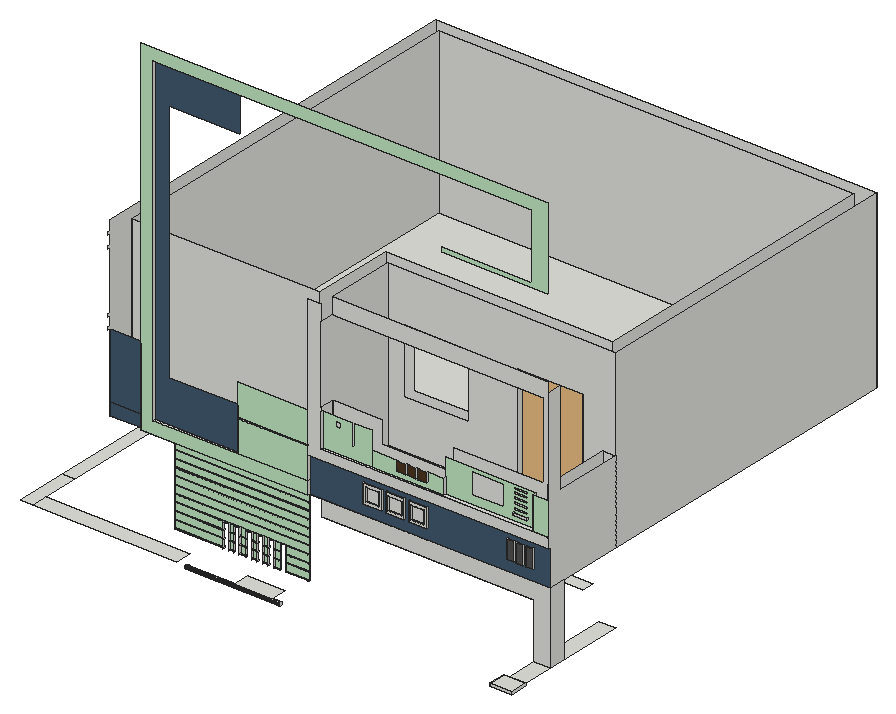
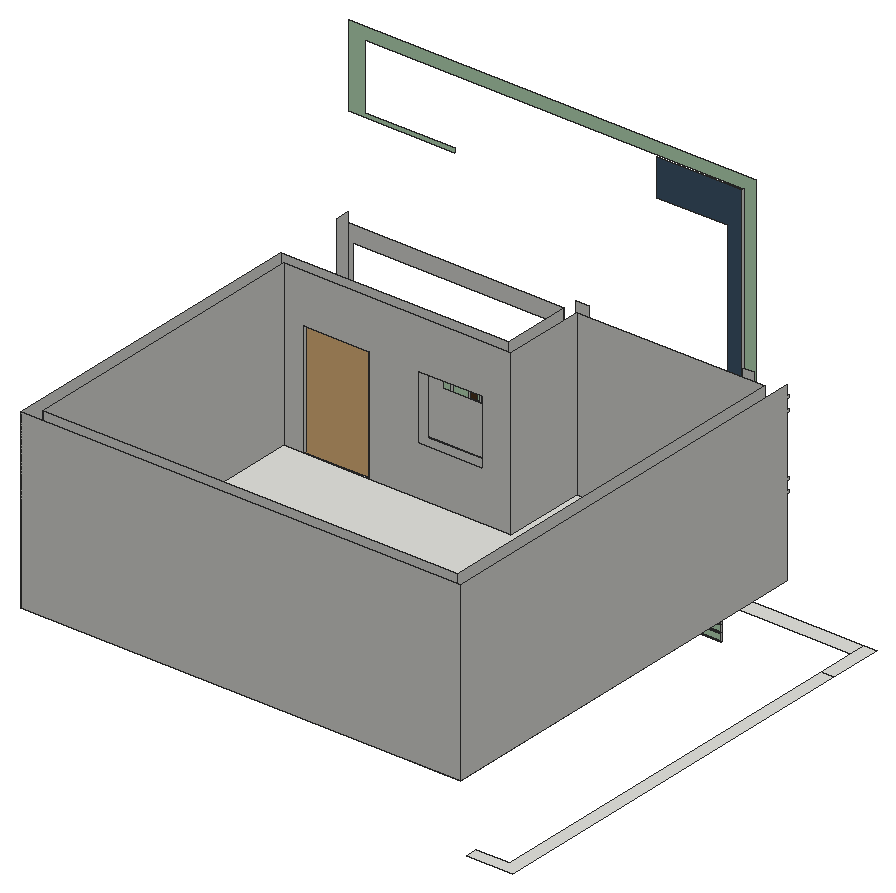
# SketchUp Ruby script. Lengths in inches.
U = 1.inch
M = Sketchup.active_model
def pt(a) = Geom::Point3d.new(a.map { |v| v * U })
def face(e, loops, mat)
  f = e.add_face(loops[0].map { |a| pt(a) })
  loops[1..].each { |l| e.add_face(l.map { |a| pt(a) }).erase! }
  f.material = f.back_material = mat if mat
  f
end
# faces: each face lists its corners as indices into pts; further lists are holes
def faces(e, pts, list, mat = nil) = list.each { |f| face(e, (f[0].is_a?(Array) ? f : [f]).map { |l| l.map { |i| pts[i] } }, mat) }
# xy, xz, yz: faces in a plane at the given z, y or x. An outline is a flat list of corners, or four numbers for a rectangle; further outlines are holes
def ring(l) = l.size == 4 ? [[l[0], l[1]], [l[2], l[1]], [l[2], l[3]], [l[0], l[3]]] : l.each_slice(2).to_a
def flat(e, list, mat, &to3) = list.each { |f| face(e, (f[0].is_a?(Array) ? f : [f]).map { |l| ring(l).map { |u, v| to3.(u, v) } }, mat) }
def xy(e, z, list, mat = nil) = flat(e, list, mat) { |x, y| [x, y, z] }
def xz(e, y, list, mat = nil) = flat(e, list, mat) { |x, z| [x, y, z] }
def yz(e, x, list, mat = nil) = flat(e, list, mat) { |y, z| [x, y, z] }
def lines(e, pts, list) = list.each { |a, b| e.add_line(pt(pts[a]), pt(pts[b])) }
# prism: a flat outline (further loops are holes) pulled along v
def prism(e, loops, v, mat = nil)
  f = face(e, loops, mat); d = Geom::Vector3d.new(v.map { |x| x * U })
  f.pushpull(f.normal.samedirection?(d) ? d.length : -d.length)
end
def box(e, o, s, mat = nil) = prism(e, [[o, [o[0] + s[0], o[1], o[2]], [o[0] + s[0], o[1] + s[1], o[2]], [o[0], o[1] + s[1], o[2]]]], [0, 0, s[2]], mat)
def at(x, y, z, deg = 0) = Geom::Transformation.translation(pt([x, y, z])) * Geom::Transformation.rotation(ORIGIN, Z_AXIS, deg.degrees)
def axes(o, x, y, z) = Geom::Transformation.new([*x, 0, *y, 0, *z, 0, *pt(o).to_a, 1])
def part(name) = M.definitions.add(name)
# library, detail: a bought-in or finely detailed component or shape, given as its bounding box
def library(name, o, s) = part(name).tap { |d| box(d.entities, o, s) }
def detail(e, o, s) = box(e.add_group.entities, o, s)
def put(e, d, t, mat = nil) = e.add_instance(d, t).tap { |i| i.material = mat if mat }
def group(e, t, mat = nil) = e.add_group.tap { |g| g.transformation = t; g.material = mat if mat }.entities
root = M.entities
M.materials.add("Teddy_SkinShadow ").color = [76, 52, 30]
M.materials.add("[0111_SlateGray]").color = [66, 89, 112]
M.materials.add("[0116_Lavender]").color = [195, 232, 195]
M.materials.add("[0135_DarkGray]1").color = [81, 81, 81]
c1 = library("porta 4",[0.2,-5.42,1.33],[46.55,4.72,83.21])
xy(root,62.5,[[131.18,38.4375,135.87,39],[83,38.5,119.37,39],[140.12,38.5,144.12,39],[148.37,38.5,152.12,39],[156.37,38.5,160.62,39],
  [164.87,38.5,182,39],[123.62,38.625,126.93,39]])
xy(root,63.25,[[83,38.5,119.37,39],[131.18,38.5,135.87,39],[140.12,38.5,144.12,39],[148.37,38.5,152.12,39],[156.37,38.5,160.62,39],
  [164.87,38.5,182,39],[123.62,38.625,126.93,39]])
xy(root,67,[[345,1,361,3],[345,3,347,12],[347,3,359,14],[359,3,361,14],[345,12,347,14],
  [347,14,359,39],[347,51,359,99]])
xy(root,68.25,[[83,38.5,119.37,39],[131.18,38.5,135.87,39],[140.12,38.5,144.12,39],[148.37,38.5,152.12,39],[156.37,38.5,160.62,39],
  [164.87,38.5,182,39],[123.62,38.625,126.93,39]])
xy(root,69,[[0,0,9,39],[9,0,115.21,12],[157.75,0,185.01,12],[345,1,361,14],[83,38.5,119.37,39],
  [131.18,38.5,135.87,39],[140.12,38.5,144.12,39],[148.37,38.5,152.12,39],[156.37,38.5,160.62,39],[164.87,38.5,182,39],
  [123.62,38.625,126.93,39],[0,39,9,39,9,325.8,34,325.8,34,334.8,0,334.8]])
xy(root,74,[[83,38.5,119.37,39],[131.18,38.5,135.87,39],[140.12,38.5,144.12,39],[148.37,38.5,152.12,39],[156.37,38.5,160.62,39],
  [164.87,38.5,182,39],[123.62,38.625,126.93,39]])
xy(root,74.75,[[83,38.5,119.37,39],[123.62,38.5,126.93,39],[131.18,38.5,135.87,39],[140.12,38.5,144.12,39],[148.37,38.5,152.12,39],
  [156.37,38.5,160.62,39],[164.87,38.5,182,39]])
xy(root,79.75,[[83,38.5,119.37,39],[164.87,38.5,182,39]])
xy(root,80.25,[[126.93,37.375,131.18,39],[135.87,37.4375,140.12,39],[144.12,37.4375,148.37,39],[119.37,37.5625,123.62,39],[152.12,37.875,156.37,39],
  [123.62,38.5,126.93,39],[131.18,38.5,135.87,39],[140.12,38.5,144.12,39],[148.37,38.5,152.12,39],[156.37,38.5,160.62,39]])
xy(root,80.5,[[83,38.5,119.37,39],[119.37,38.5,164.87,39],[164.87,38.5,182,39]])
xy(root,84,[[203,99,251,108],[287,99,335,108]])
xy(root,85.5,[[83,38.5,119.37,39],[119.37,38.5,164.87,39],[164.87,38.5,182,39]])
xy(root,86.25,[[83,38.5,119.37,39],[119.37,38.5,164.87,39],[164.87,38.5,182,39]])
xy(root,91.25,[[83,38.5,119.37,39],[119.37,38.5,164.87,39],[164.87,38.5,182,39]])
xy(root,92,[[83,38.5,119.37,39],[119.37,38.5,164.87,39],[164.87,38.5,182,39]])
xy(root,97,[[83,38.5,119.37,39],[119.37,38.5,164.87,39],[164.87,38.5,182,39]])
xy(root,97.75,[[83,38.5,119.37,39],[119.37,38.5,164.87,39],[164.87,38.5,182,39]])
xy(root,102.75,[[83,38.5,119.37,39],[119.37,38.5,164.87,39],[164.87,38.5,182,39]])
xy(root,103.5,[[83,38.5,119.37,39],[119.37,38.5,164.87,39],[164.87,38.5,182,39]])
xy(root,108,[[191,39,347,51]])
xy(root,108.5,[[83,38.5,119.37,39],[119.37,38.5,164.87,39],[164.87,38.5,182,39]])
xy(root,109.25,[[83,38.5,119.37,39],[119.37,38.5,164.87,39],[164.87,38.5,182,39]])
xy(root,114.25,[[83,38.5,119.37,39],[119.37,38.5,164.87,39],[164.87,38.5,182,39]])
xy(root,115,[[83,38.5,119.37,39],[119.37,38.5,164.87,39],[164.87,38.5,182,39]])
xy(root,120,[[59,37,59,39,83,39,83,38.5,182,38.5,182,37],[83,38.5,182,39],[35,39,44,339],[44,39,83,48],[83,39,92,99],
  [92,39,92,48,182,48,182,90,92,90,92,99,191,99,191,39],[191,39,359,51],[44,48,83,330],[92,48,182,90],[191,51,359,99],
  [83,99,92,108],[92,99,359,99,359,339,92,339,92,330,350,330,350,108,92,108],[83,108,92,339],[92,108,350,330],[44,330,83,339]])
xy(root,127.88,[[221.83,38,235.58,39],[238.46,38,252.21,39],[255.27,38,269.02,39]])
xy(root,128.49,[[327.94,38,332.88,39],[334.69,38,339.63,39],[342,38,346.94,39]])
xy(root,129,[[68,37,182,37,182,37.5,130.11,37.5,130.11,39,68,39],[130.11,37.5,182,39],[44,48,182.375,48,182.375,108,350,108,350,330,44,330],[191.375,48,350,48,350,99,334.8125,99,334.8125,108,287,108,287,99,191.375,99]])
xy(root,129.88,[[223.83,38,233.58,39],[240.46,38,250.21,39],[257.27,38,267.02,39]])
xy(root,139.63,[[223.83,38,233.58,39],[240.46,38,250.21,39],[257.27,38,267.02,39]])
xy(root,141.63,[[221.83,38,235.58,39],[238.46,38,252.21,39],[255.27,38,269.02,39]])
xy(root,141.87,[[327.94,38,332.88,39],[334.69,38,339.63,39],[342,38,346.94,39]])
xy(root,146.25,[[182,37.5,359,39]])
xy(root,152,[[130.11,37.5,182,39]])
xy(root,153,[[130.11,37.5,182,39]])
xy(root,153.78,[[191.375,37.5,227.375,39],[227.375,37.5,280.75,39],[280.75,37.5,359,37.5,359,38,347,38,347,40.75,280.75,40.75]])
xy(root,157.71,[[330.79,39.75,341.29,40.75]])
xy(root,158.06,[[247.03,38,253.34,39],[254.72,38,261.03,39],[262.4,38,268.72,39]])
xz(root,1,[[345,67,361,69]])
xz(root,14,[[345,67,361,69]])
xz(root,37,[[59,120,182,120,182,129,68,129,68,366,347,366,347,318,280.59,318,280.59,315,359,315,359,375,59,375]],"[0116_Lavender]")
xz(root,37.5,[[182,146.25,359,146.25,359,153.78,191.375,153.78,191.375,249,182,249]])
xz(root,37.5,[[130.11,129,182,152],[130.11,153,182,176]],"[0116_Lavender]")
xz(root,38,[[[221.83,127.88,235.58,141.63],[223.83,129.88,233.58,139.63]],[[238.46,127.88,252.21,141.63],[240.46,129.88,250.21,139.63]],[[255.27,127.88,269.02,141.63],[257.27,129.88,267.02,139.63]]])
xz(root,38,[[247.03,158.06,253.34,164.72],[254.72,158.06,261.03,164.72],[262.4,158.06,268.72,164.72]],"Teddy_SkinShadow ")
xz(root,38,[[347,153.78,359,177.875]],"[0116_Lavender]")
xz(root,38,[[327.94,128.49,332.88,141.87],[334.69,128.49,339.63,141.87],[342,128.49,346.94,141.87]],"[0135_DarkGray]1")
xz(root,38.5,[[83,63.25,119.37,68.25],[131.18,63.25,135.87,68.25],[140.12,63.25,144.12,68.25],[148.37,63.25,152.12,68.25],[156.37,63.25,160.62,68.25],
  [164.87,63.25,182,68.25],[83,69,119.37,74],[131.18,69,135.87,74],[140.12,69,144.12,74],[148.37,69,152.12,74],
  [156.37,69,160.62,74],[164.87,69,182,74],[83,74.75,119.37,79.75],[123.62,74.75,126.93,80.25],[131.18,74.75,135.87,80.25],
  [140.12,74.75,144.12,80.25],[148.37,74.75,152.12,80.25],[156.37,74.75,160.62,80.25],[164.87,74.75,182,79.75],[83,80.5,182,85.5],
  [83,86.25,182,91.25],[83,92,182,97],[83,97.75,182,102.75],[83,103.5,182,108.5],[83,109.25,182,114.25],
  [83,115,182,120]],"[0116_Lavender]")
xz(root,38.625,[[123.62,63.25,126.93,68.25],[123.62,69,126.93,74]],"[0116_Lavender]")
xz(root,39,[[83,62.5,119.37,63.25],[123.62,62.5,126.93,63.25],[131.18,62.5,135.87,63.25],[140.12,62.5,144.12,63.25],[148.37,62.5,152.12,63.25],
  [156.37,62.5,160.62,63.25],[164.87,62.5,182,63.25],[347,67,359,67,359,120,191,120,191,108,347,108],[83,68.25,119.37,69],[123.62,68.25,126.93,69],
  [131.18,68.25,135.87,69],[140.12,68.25,144.12,69],[148.37,68.25,152.12,69],[156.37,68.25,160.62,69],[83,74,119.37,74.75],
  [123.62,74,126.93,74.75],[131.18,74,135.87,74.75],[140.12,74,144.12,74.75],[148.37,74,152.12,74.75],[156.37,74,160.62,74.75],
  [164.87,74,182,74.75],[83,79.75,119.37,79.75,119.37,80.25,164.87,80.25,164.87,79.75,182,79.75,182,80.5,83,80.5],[83,85.5,182,86.25],[83,91.25,182,92],[83,97,182,97.75],
  [83,102.75,182,103.5],[83,108.5,182,109.25],[83,114.25,182,115],[83,115,182,120],[59,120,182,129],
  [59,129,68,249],[223.83,129.88,233.58,139.63],[240.46,129.88,250.21,139.63],[257.27,129.88,267.02,139.63],[130.11,152,182,153]])
xz(root,39,[[35,120,59,129],[[182,120,359,146.25],[221.83,127.88,235.58,141.63],[238.46,127.88,252.21,141.63],[255.27,127.88,269.02,141.63],[327.94,128.49,332.88,141.87],[334.69,128.49,339.63,141.87],[342,128.49,346.94,141.87]],[35,129,59,177.03],[68,129,130.11,129,130.11,160.2,78.11,160.2,78.11,339.39,130.11,339.39,130.11,366,68,366]],"[0111_SlateGray]")
xz(root,39,[[164.87,68.25,182,69],[[191.375,153.78,227.375,153.78,227.375,177.875,215.16,177.875,215.16,162.5625,212.91,162.5625,212.91,177.875,191.375,177.875],[201.03,170.65,204.85,174.46]],[227.375,153.78,280.75,153.78,280.75,164.72,268.72,164.72,268.72,158.06,262.4,158.06,262.4,164.72,261.03,164.72,261.03,158.06,254.72,158.06,254.72,164.72,253.34,164.72,253.34,158.06,247.03,158.06,247.03,164.72,227.375,164.72]],"[0116_Lavender]")
xz(root,39.75,[[330.79,157.71,341.29,159.46]])
xz(root,40.75,[[[280.75,153.78,347,177.875],[299.99,160.18,323.67,175.49],[330.79,174.4,341.29,176.15],[330.79,171.46,341.29,173.21],[330.79,168.15,341.29,169.9],[330.79,164.71,341.29,166.46],[330.79,160.9,341.29,162.65],[330.79,157.71,341.29,159.46]]],"[0116_Lavender]")
xz(root,48,[[44,129,182.375,249],[191.375,129,191.375,180.875,227.375,180.875,227.375,164.72,280.75,164.72,280.75,180.875,347,180.875,347,237,191.375,237,191.375,249,350,249,350,129]])
xz(root,51,[[347,67,347,108,191,108,191,120,359,120,359,67]])
xz(root,99,[[[191.375,129,287,129,287,213,334.8125,213,334.8125,129,350,129,350,180.875,359,180.875,359,249,191.375,249],[203,165,251,213]]])
xz(root,108,[[[182.375,129,182.375,249,350,249,350,129,334.8125,129,334.8125,213,287,213,287,129],[203,165,251,213]]])
xz(root,330,[[44,129,350,249]])
xz(root,339,[[35,120,359,249]])
yz(root,35,[[39,120,39,177.03,37,177.03,37,179.03,39,179.03,39,185.53,37,185.53,37,187.53,39,187.53,39,230.47,37,230.47,37,232.47,39,232.47,39,239.9,37,239.9,37,241.9,39,241.9,39,249,339,249,339,120]])
yz(root,44,[[48,129,330,249]])
yz(root,59,[[37,120,39,177.03]])
yz(root,68,[[37,129,39,366]])
yz(root,83,[[38.5,63.25,39,68.25],[38.5,69,39,74],[38.5,74.75,39,79.75],[38.5,80.5,39,85.5],[38.5,86.25,39,91.25],
  [38.5,92,39,97],[38.5,97.75,39,102.75],[38.5,103.5,39,108.5],[38.5,109.25,39,114.25],[38.5,115,39,120]])
yz(root,119.37,[[37.5625,62.5,39,63.25],[37.5625,63.25,38.5,68.25],[37.5625,68.25,39,69],[37.5625,69,38.5,74],[37.5625,74,39,74.75],
  [37.5625,74.75,38.5,79.75],[37.5625,79.75,39,80.25]])
yz(root,123.62,[[37.5625,62.5,39,63.25],[37.5625,63.25,38.625,68.25],[37.5625,68.25,39,69],[37.5625,69,38.625,74],[37.5625,74,39,74.75],
  [37.5625,74.75,38.5,80.25]])
yz(root,126.93,[[37.375,62.5,39,63.25],[37.375,63.25,38.625,68.25],[37.375,68.25,39,69],[37.375,69,38.625,74],[37.375,74,39,74.75],
  [37.375,74.75,38.5,80.25]])
yz(root,130.11,[[37.5,129,39,152],[37.5,153,39,160.2]])
yz(root,131.18,[[37.375,62.5,39,63.25],[37.375,63.25,38.5,68.25],[37.375,68.25,39,69],[37.375,69,38.5,74],[37.375,74,39,74.75],
  [37.375,74.75,38.5,80.25]])
yz(root,135.87,[[37.4375,62.5,39,63.25],[37.4375,63.25,38.5,68.25],[37.4375,68.25,39,69],[37.4375,69,38.5,74],[37.4375,74,39,74.75],
  [37.4375,74.75,38.5,80.25]])
yz(root,140.12,[[37.4375,62.5,39,63.25],[37.4375,63.25,38.5,68.25],[37.4375,68.25,39,69],[37.4375,69,38.5,74],[37.4375,74,39,74.75],
  [37.4375,74.75,38.5,80.25]])
yz(root,144.12,[[37.4375,62.5,39,63.25],[37.4375,63.25,38.5,68.25],[37.4375,68.25,39,69],[37.4375,69,38.5,74],[37.4375,74,39,74.75],
  [37.4375,74.75,38.5,80.25]])
yz(root,148.37,[[37.4375,62.5,39,63.25],[37.4375,63.25,38.5,68.25],[37.4375,68.25,39,69],[37.4375,69,38.5,74],[37.4375,74,39,74.75],
  [37.4375,74.75,38.5,80.25]])
yz(root,152.12,[[37.875,62.5,39,63.25],[37.875,63.25,38.5,68.25],[37.875,68.25,39,69],[37.875,69,38.5,74],[37.875,74,39,74.75],
  [37.875,74.75,38.5,80.25]])
yz(root,156.37,[[37.875,62.5,39,63.25],[37.875,63.25,38.5,68.25],[37.875,68.25,39,69],[37.875,69,38.5,74],[37.875,74,39,74.75],
  [37.875,74.75,38.5,80.25]])
yz(root,160.62,[[38.5,63.25,39,68.25],[38.5,69,39,74],[38.5,74.75,39,80.25]])
yz(root,164.87,[[38.5,63.25,39,68.25],[38.5,69,39,74],[38.5,74.75,39,79.75]])
yz(root,182,[[38.5,63.25,39,68.25],[38.5,69,39,74],[38.5,74.75,39,79.75],[38.5,80.5,39,85.5],[38.5,86.25,39,91.25],
  [38.5,92,39,97],[38.5,97.75,39,102.75],[38.5,103.5,39,108.5],[38.5,109.25,39,114.25],[38.5,115,39,120],
  [37,120,39,129],[37.5,129,39,146.25],[37.5,152,39,153]])
yz(root,182.375,[[48,129,108,249]])
yz(root,184.86,[[8.625,60.67,8.92,60.71,9.1875,60.82,9.42,61,9.6,61.24,9.71,61.51,9.75,61.8,9.71,62.09,9.6,62.36,9.42,62.59,9.1875,62.77,8.92,62.88,8.625,62.92,8.33,62.88,8.0625,62.77,7.83,62.59,7.65,62.36,7.54,62.09,7.5,61.8,7.54,61.51,7.65,61.24,7.83,61,8.0625,60.82,8.33,60.71]])
yz(root,191.375,[[48,129,99,129,99,249,49.5,249,49.5,237,37.5,237,37.5,180.875,48,180.875],[37.5,153.78,39,177.875]])
yz(root,221.83,[[38,127.88,39,141.63]])
yz(root,223.83,[[38,129.88,39,139.63]])
yz(root,233.58,[[38,129.88,39,139.63]])
yz(root,235.58,[[38,127.88,39,141.63]])
yz(root,238.46,[[38,127.88,39,141.63]])
yz(root,240.46,[[38,129.88,39,139.63]])
yz(root,247.03,[[38,158.06,39,159.43]])
yz(root,250.21,[[38,129.88,39,139.63]])
yz(root,252.21,[[38,127.88,39,141.63]])
yz(root,253.34,[[38,158.06,39,164.72]])
yz(root,254.72,[[38,158.06,39,159.43]])
yz(root,255.27,[[38,127.88,39,141.63]])
yz(root,257.27,[[38,129.88,39,139.63]])
yz(root,261.03,[[38,158.06,39,164.72]])
yz(root,262.4,[[38,158.06,39,159.43]])
yz(root,267.02,[[38,129.88,39,139.63]])
yz(root,268.72,[[38,158.06,39,164.72]])
yz(root,269.02,[[38,127.88,39,141.63]])
yz(root,280.75,[[39,153.78,40.75,164.72]])
yz(root,287,[[99,129,108,213]])
yz(root,327.94,[[38,128.49,39,141.87]])
yz(root,330.79,[[39.75,157.71,40.75,159.46]])
yz(root,332.88,[[38,128.49,39,141.87]])
yz(root,334.69,[[38,128.49,39,141.87]])
yz(root,334.8125,[[99,129,108,213]])
yz(root,339.63,[[38,128.49,39,141.87]])
yz(root,341.29,[[39.75,157.71,40.75,159.46]])
yz(root,342,[[38,128.49,39,141.87]])
yz(root,345,[[1,67,14,69]])
yz(root,346.94,[[38,128.49,39,141.87]])
yz(root,347,[[38,153.78,40.75,177.875]])
yz(root,350,[[48,129,99,180.875],[108,129,330,249]])
yz(root,359,[[39,67,51,120],[39,120,99,120,99,180.875,48,180.875,48,249,38,249,38,153.78,37.5,153.78,37.5,146.25,39,146.25],[99,120,339,249]])
yz(root,361,[[1,67,14,69]])
p = [[115.21,8.0625,60.82],[115.21,8.33,60.71],[184.86,8.33,60.71],[184.86,8.0625,60.82],[115.21,8.625,60.67],[184.86,8.625,60.67],
  [115.21,8.92,60.71],[184.86,8.92,60.71],[115.21,9.1875,60.82],[184.86,9.1875,60.82],[115.21,7.83,61],[184.86,7.83,61],
  [115.21,9.42,61],[184.86,9.42,61],[115.21,7.65,61.24],[184.86,7.65,61.24],[115.21,9.6,61.24],[184.86,9.6,61.24],
  [115.21,7.54,61.51],[184.86,7.54,61.51],[115.21,9.71,61.51],[184.86,9.71,61.51],[115.21,7.5,61.8],[184.86,7.5,61.8],
  [115.21,9.75,61.8],[184.86,9.75,61.8],[115.21,7.54,62.09],[184.86,7.54,62.09],[115.21,9.71,62.09],[184.86,9.71,62.09],
  [115.21,7.65,62.36],[184.86,7.65,62.36],[115.21,9.6,62.36],[184.86,9.6,62.36],[115.21,7.83,62.59],[184.86,7.83,62.59],
  [115.21,9.42,62.59],[184.86,9.42,62.59],[115.21,8.0625,62.77],[184.86,8.0625,62.77],[115.21,9.1875,62.77],[184.86,9.1875,62.77],
  [115.21,8.33,62.88],[184.86,8.33,62.88],[115.21,8.92,62.88],[184.86,8.92,62.88],[115.21,8.625,62.92],[184.86,8.625,62.92]]
faces(root,p,[[0,1,2,3],[1,4,5,2],[4,6,7,5],[6,8,9,7],[10,0,3,11],[8,12,13,9],[14,10,11,15],[12,16,17,13],
  [18,14,15,19],[16,20,21,17],[22,18,19,23],[20,24,25,21],[26,22,23,27],[24,28,29,25],[30,26,27,31],[28,32,33,29],
  [34,30,31,35],[32,36,37,33],[38,34,35,39],[36,40,41,37],[42,38,39,43],[40,44,45,41],[46,42,43,47],[44,46,47,45]])
put(root,c1,axes([286.79,107.51,127.64],[1.03092,0,0],[0,0.9372,0],[0,0,1.01218]))
